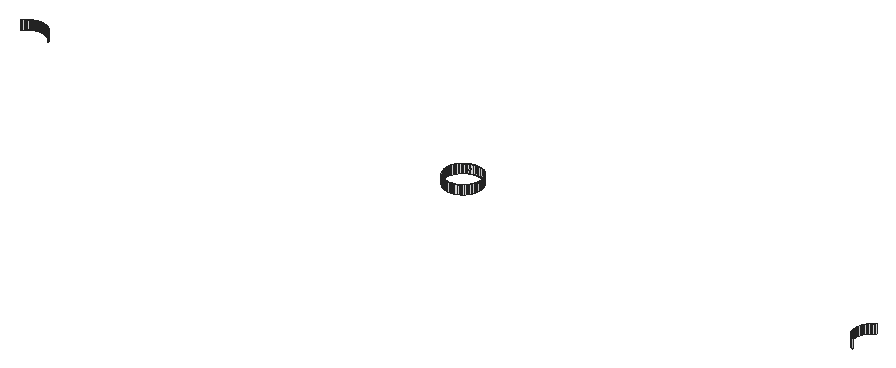
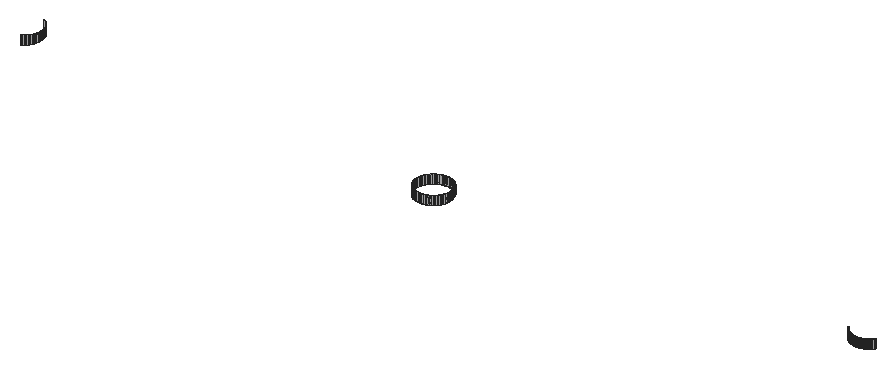
# SketchUp Ruby script. Lengths in inches.
U = 1.inch
M = Sketchup.active_model
def pt(a) = Geom::Point3d.new(a.map { |v| v * U })
def face(e, loops, mat)
  f = e.add_face(loops[0].map { |a| pt(a) })
  loops[1..].each { |l| e.add_face(l.map { |a| pt(a) }).erase! }
  f.material = f.back_material = mat if mat
  f
end
# faces: each face lists its corners as indices into pts; further lists are holes
def faces(e, pts, list, mat = nil) = list.each { |f| face(e, (f[0].is_a?(Array) ? f : [f]).map { |l| l.map { |i| pts[i] } }, mat) }
# xy, xz, yz: faces in a plane at the given z, y or x. An outline is a flat list of corners, or four numbers for a rectangle; further outlines are holes
def ring(l) = l.size == 4 ? [[l[0], l[1]], [l[2], l[1]], [l[2], l[3]], [l[0], l[3]]] : l.each_slice(2).to_a
def flat(e, list, mat, &to3) = list.each { |f| face(e, (f[0].is_a?(Array) ? f : [f]).map { |l| ring(l).map { |u, v| to3.(u, v) } }, mat) }
def xy(e, z, list, mat = nil) = flat(e, list, mat) { |x, y| [x, y, z] }
def xz(e, y, list, mat = nil) = flat(e, list, mat) { |x, z| [x, y, z] }
def yz(e, x, list, mat = nil) = flat(e, list, mat) { |y, z| [x, y, z] }
def lines(e, pts, list) = list.each { |a, b| e.add_line(pt(pts[a]), pt(pts[b])) }
# prism: a flat outline (further loops are holes) pulled along v
def prism(e, loops, v, mat = nil)
  f = face(e, loops, mat); d = Geom::Vector3d.new(v.map { |x| x * U })
  f.pushpull(f.normal.samedirection?(d) ? d.length : -d.length)
end
def box(e, o, s, mat = nil) = prism(e, [[o, [o[0] + s[0], o[1], o[2]], [o[0] + s[0], o[1] + s[1], o[2]], [o[0], o[1] + s[1], o[2]]]], [0, 0, s[2]], mat)
def at(x, y, z, deg = 0) = Geom::Transformation.translation(pt([x, y, z])) * Geom::Transformation.rotation(ORIGIN, Z_AXIS, deg.degrees)
def axes(o, x, y, z) = Geom::Transformation.new([*x, 0, *y, 0, *z, 0, *pt(o).to_a, 1])
def part(name) = M.definitions.add(name)
# library, detail: a bought-in or finely detailed component or shape, given as its bounding box
def library(name, o, s) = part(name).tap { |d| box(d.entities, o, s) }
def detail(e, o, s) = box(e.add_group.entities, o, s)
def put(e, d, t, mat = nil) = e.add_instance(d, t).tap { |i| i.material = mat if mat }
def group(e, t, mat = nil) = e.add_group.tap { |g| g.transformation = t; g.material = mat if mat }.entities
root = M.entities
M.materials.add("[Quartz Light Grey]").color = [251, 251, 252]
xz(root,225.96,[[38.36,111.81,38.38,112.81],[39.62,111.81,39.64,112.81]],"[Quartz Light Grey]")
xz(root,226.01,[[38.52,111.81,38.5625,112.81],[39.4375,111.81,39.48,112.81]],"[Quartz Light Grey]")
xz(root,226.03,[[38.625,111.81,38.65,112.81],[39.35,111.81,39.375,112.81]],"[Quartz Light Grey]")
xz(root,226.04,[[38.6875,111.81,38.73,112.81],[39.27,111.81,39.3125,112.81]],"[Quartz Light Grey]")
xz(root,226.05,[[38.75,111.81,38.77,112.81],[38.77,111.81,38.8125,112.81],[39.1875,111.81,39.23,112.81],[39.23,111.81,39.25,112.81]],"[Quartz Light Grey]")
xz(root,226.06,[[38.85,111.81,38.875,112.81],[38.875,111.81,38.9,112.81],[39.1,111.81,39.125,112.81],[39.125,111.81,39.15,112.81]],"[Quartz Light Grey]")
xz(root,226.0625,[[38.9375,111.81,38.98,112.81],[38.98,111.81,39,112.81],[39,111.81,39.02,112.81],[39.02,111.81,39.0625,112.81]],"[Quartz Light Grey]")
yz(root,85,[[227.96,111.81,228.08,112.81]],"[Quartz Light Grey]")
yz(root,89,[[228.04,111.81,228.17,112.81]],"[Quartz Light Grey]")
yz(root,133,[[227.96,111.81,228.08,112.81]],"[Quartz Light Grey]")
p = [[40.72,225.08,111.81],[40.74,225.05,111.81],[40.74,225.05,112.81],[40.72,225.08,112.81],[40.68,225.15,111.81],[40.6875,225.13,111.81],
  [40.6875,225.13,112.81],[40.68,225.15,112.81],[40.7,225.12,111.81],[40.7,225.12,112.81],[37.35,225.1875,111.81],[37.37,225.22,111.81],
  [37.37,225.22,112.81],[37.35,225.1875,112.81],[37.38,225.24,111.81],[37.38,225.24,112.81],[37.39,225.26,111.81],[37.39,225.26,112.81],
  [40.61,225.26,111.81],[40.62,225.24,111.81],[40.62,225.24,112.81],[40.61,225.26,112.81],[40.63,225.22,111.81],[40.63,225.22,112.81],
  [40.65,225.1875,111.81],[40.65,225.1875,112.81],[37.42,225.29,111.81],[37.42,225.29,112.81],[37.45,225.32,111.81],[37.45,225.32,112.81],
  [37.46,225.34,111.81],[37.46,225.34,112.81],[37.47,225.35,111.81],[37.47,225.35,112.81],[40.53,225.35,111.81],[40.54,225.34,111.81],
  [40.54,225.34,112.81],[40.53,225.35,112.81],[40.55,225.32,111.81],[40.55,225.32,112.81],[40.58,225.29,111.81],[40.58,225.29,112.81],
  [37.5,225.38,111.81],[37.5,225.38,112.81],[37.53,225.42,111.81],[37.53,225.42,112.81],[37.54,225.43,111.81],[37.54,225.43,112.81],
  [37.56,225.45,111.81],[37.56,225.45,112.81],[37.59,225.48,111.81],[37.59,225.48,112.81],[40.41,225.48,111.81],[40.44,225.45,111.81],
  [40.44,225.45,112.81],[40.41,225.48,112.81],[40.46,225.43,111.81],[40.46,225.43,112.81],[40.47,225.42,111.81],[40.47,225.42,112.81],
  [40.5,225.38,111.81],[40.5,225.38,112.81],[37.62,225.51,111.81],[37.62,225.51,112.81],[37.63,225.52,111.81],[37.63,225.52,112.81],
  [37.65,225.54,111.81],[37.65,225.54,112.81],[37.68,225.5625,111.81],[37.68,225.5625,112.81],[40.32,225.5625,111.81],[40.35,225.54,111.81],
  [40.35,225.54,112.81],[40.32,225.5625,112.81],[40.37,225.52,111.81],[40.37,225.52,112.81],[40.38,225.51,111.81],[40.38,225.51,112.81],
  [37.71,225.59,111.81],[37.71,225.59,112.81],[37.73,225.6,111.81],[37.73,225.6,112.81],[37.74,225.62,111.81],[37.74,225.62,112.81],
  [37.77,225.64,111.81],[37.77,225.64,112.81],[37.81,225.67,111.81],[37.81,225.67,112.81],[40.19,225.67,111.81],[40.23,225.64,111.81],
  [40.23,225.64,112.81],[40.19,225.67,112.81],[40.26,225.62,111.81],[40.26,225.62,112.81],[40.27,225.6,111.81],[40.27,225.6,112.81],
  [40.29,225.59,111.81],[40.29,225.59,112.81],[37.82,225.68,111.81],[37.82,225.68,112.81],[37.84,225.69,111.81],[37.84,225.69,112.81],
  [37.875,225.72,111.81],[37.875,225.72,112.81],[37.91,225.74,111.81],[37.91,225.74,112.81],[37.93,225.75,111.81],[37.93,225.75,112.81],
  [40.07,225.75,111.81],[40.09,225.74,111.81],[40.09,225.74,112.81],[40.07,225.75,112.81],[40.125,225.72,111.81],[40.125,225.72,112.81],
  [40.16,225.69,111.81],[40.16,225.69,112.81],[40.18,225.68,111.81],[40.18,225.68,112.81],[37.95,225.76,111.81],[37.95,225.76,112.81],
  [37.98,225.78,111.81],[37.98,225.78,112.81],[38.02,225.8,111.81],[38.02,225.8,112.81],[38.04,225.81,111.81],[38.04,225.81,112.81],
  [38.06,225.83,111.81],[38.06,225.83,112.81],[38.09,225.84,111.81],[38.09,225.84,112.81],[38.13,225.86,111.81],[38.13,225.86,112.81],
  [39.87,225.86,111.81],[39.91,225.84,111.81],[39.91,225.84,112.81],[39.87,225.86,112.81],[39.94,225.83,111.81],[39.94,225.83,112.81],
  [39.96,225.81,111.81],[39.96,225.81,112.81],[39.98,225.8,111.81],[39.98,225.8,112.81],[40.02,225.78,111.81],[40.02,225.78,112.81],
  [40.05,225.76,111.81],[40.05,225.76,112.81],[38.15,225.87,111.81],[38.15,225.87,112.81],[38.17,225.88,111.81],[38.17,225.88,112.81],
  [38.21,225.9,111.81],[38.21,225.9,112.81],[38.24,225.91,111.81],[38.24,225.91,112.81],[38.26,225.92,111.81],[38.26,225.92,112.81],
  [38.28,225.93,111.81],[38.28,225.93,112.81],[38.32,225.94,111.81],[38.32,225.94,112.81],[38.36,225.96,111.81],[38.36,225.96,112.81],
  [39.64,225.96,111.81],[39.68,225.94,111.81],[39.68,225.94,112.81],[39.64,225.96,112.81],[39.72,225.93,111.81],[39.72,225.93,112.81],
  [39.74,225.92,111.81],[39.74,225.92,112.81],[39.76,225.91,111.81],[39.76,225.91,112.81],[39.79,225.9,111.81],[39.79,225.9,112.81],
  [39.83,225.88,111.81],[39.83,225.88,112.81],[39.85,225.87,111.81],[39.85,225.87,112.81],[38.38,225.96,111.81],[38.4,225.97,111.81],
  [38.4,225.97,112.81],[38.38,225.96,112.81],[38.44,225.98,111.81],[38.44,225.98,112.81],[38.48,225.99,111.81],[38.48,225.99,112.81],
  [38.5,226,111.81],[38.5,226,112.81],[38.52,226.01,111.81],[38.52,226.01,112.81],[38.5625,226.01,111.81],[38.6,226.02,111.81],
  [38.6,226.02,112.81],[38.5625,226.01,112.81],[38.625,226.03,111.81],[38.625,226.03,112.81],[38.65,226.03,111.81],[38.6875,226.04,111.81],
  [38.6875,226.04,112.81],[38.65,226.03,112.81],[38.73,226.04,111.81],[38.75,226.05,111.81],[38.75,226.05,112.81],[38.73,226.04,112.81],
  [39.25,226.05,111.81],[39.27,226.04,111.81],[39.27,226.04,112.81],[39.25,226.05,112.81],[39.3125,226.04,111.81],[39.35,226.03,111.81],
  [39.35,226.03,112.81],[39.3125,226.04,112.81],[39.375,226.03,111.81],[39.4,226.02,111.81],[39.4,226.02,112.81],[39.375,226.03,112.81],
  [39.4375,226.01,111.81],[39.4375,226.01,112.81],[39.48,226.01,111.81],[39.5,226,111.81],[39.5,226,112.81],[39.48,226.01,112.81],
  [39.52,225.99,111.81],[39.52,225.99,112.81],[39.56,225.98,111.81],[39.56,225.98,112.81],[39.6,225.97,111.81],[39.6,225.97,112.81],
  [39.62,225.96,111.81],[39.62,225.96,112.81],[38.8125,226.05,111.81],[38.85,226.06,111.81],[38.85,226.06,112.81],[38.8125,226.05,112.81],
  [38.9,226.06,111.81],[38.9375,226.0625,111.81],[38.9375,226.0625,112.81],[38.9,226.06,112.81],[39.0625,226.0625,111.81],[39.1,226.06,111.81],
  [39.1,226.06,112.81],[39.0625,226.0625,112.81],[39.15,226.06,111.81],[39.1875,226.05,111.81],[39.1875,226.05,112.81],[39.15,226.06,112.81],
  [86.48,226.13,111.81],[86.36,226.17,111.81],[86.36,226.17,112.81],[86.48,226.13,112.81],[86.6,226.1,111.81],[86.6,226.1,112.81],
  [86.73,226.08,111.81],[86.73,226.08,112.81],[86.85,226.07,111.81],[86.85,226.07,112.81],[86.98,226.0625,111.81],[86.98,226.0625,112.81],
  [87.1,226.07,111.81],[87.1,226.07,112.81],[87.23,226.08,111.81],[87.23,226.08,112.81],[87.35,226.09,111.81],[87.35,226.09,112.81],
  [87.48,226.12,111.81],[87.48,226.12,112.81],[87.6,226.15,111.81],[87.6,226.15,112.81],[86.24,226.21,111.81],[86.13,226.26,111.81],
  [86.13,226.26,112.81],[86.24,226.21,112.81],[87.72,226.2,111.81],[87.72,226.2,112.81],[87.83,226.24,111.81],[87.83,226.24,112.81],
  [87.94,226.3,111.81],[87.94,226.3,112.81],[86.02,226.32,111.81],[85.91,226.39,111.81],[85.91,226.39,112.81],[86.02,226.32,112.81],
  [88.05,226.36,111.81],[88.05,226.36,112.81],[134.02,226.32,111.81],[133.91,226.39,111.81],[133.91,226.39,112.81],[134.02,226.32,112.81],
  [134.13,226.26,111.81],[134.13,226.26,112.81],[85.81,226.46,111.81],[85.81,226.46,112.81],[88.16,226.43,111.81],[88.16,226.43,112.81],
  [88.26,226.51,111.81],[88.26,226.51,112.81],[133.81,226.46,111.81],[133.81,226.46,112.81],[85.71,226.54,111.81],[85.62,226.62,111.81],
  [85.62,226.62,112.81],[85.71,226.54,112.81],[88.35,226.59,111.81],[88.35,226.59,112.81],[133.71,226.54,111.81],[133.62,226.62,111.81],
  [133.62,226.62,112.81],[133.71,226.54,112.81],[85.53,226.71,111.81],[85.53,226.71,112.81],[88.44,226.68,111.81],[88.44,226.68,112.81],
  [133.53,226.71,111.81],[133.53,226.71,112.81],[85.45,226.8,111.81],[85.45,226.8,112.81],[88.53,226.77,111.81],[88.53,226.77,112.81],
  [133.45,226.8,111.81],[133.45,226.8,112.81],[85.37,226.9,111.81],[85.37,226.9,112.81],[88.61,226.87,111.81],[88.61,226.87,112.81],
  [133.37,226.9,111.81],[133.37,226.9,112.81],[85.3,227.01,111.81],[85.3,227.01,112.81],[88.68,226.97,111.81],[88.68,226.97,112.81],
  [133.3,227.01,111.81],[133.3,227.01,112.81],[85.24,227.12,111.81],[85.24,227.12,112.81],[88.74,227.08,111.81],[88.74,227.08,112.81],
  [133.24,227.12,111.81],[133.24,227.12,112.81],[85.18,227.23,111.81],[85.18,227.23,112.81],[88.8,227.19,111.81],[88.8,227.19,112.81],
  [133.18,227.23,111.81],[133.18,227.23,112.81],[85.13,227.35,111.81],[85.13,227.35,112.81],[88.85,227.31,111.81],[88.85,227.31,112.81],
  [133.13,227.35,111.81],[133.13,227.35,112.81],[85.09,227.47,111.81],[85.09,227.47,112.81],[88.9,227.42,111.81],[88.9,227.42,112.81],
  [133.09,227.47,111.81],[133.09,227.47,112.81],[88.93,227.54,111.81],[88.93,227.54,112.81],[85.06,227.59,111.81],[85.06,227.59,112.81],
  [88.96,227.67,111.81],[88.96,227.67,112.81],[133.06,227.59,111.81],[133.06,227.59,112.81],[85.03,227.71,111.81],[85.03,227.71,112.81],
  [133.03,227.71,111.81],[133.03,227.71,112.81],[85.01,227.83,111.81],[85.01,227.83,112.81],[88.98,227.79,111.81],[88.98,227.79,112.81],
  [133.01,227.83,111.81],[133.01,227.83,112.81],[85,227.96,111.81],[85,227.96,112.81],[88.99,227.92,111.81],[88.99,227.92,112.81],
  [133,227.96,111.81],[133,227.96,112.81],[89,228.04,111.81],[89,228.04,112.81],[85,228.08,111.81],[85.01,228.21,111.81],
  [85.01,228.21,112.81],[85,228.08,112.81],[133,228.08,111.81],[133.01,228.21,111.81],[133.01,228.21,112.81],[133,228.08,112.81],
  [85.02,228.33,111.81],[85.02,228.33,112.81],[88.99,228.29,111.81],[89,228.17,111.81],[89,228.17,112.81],[88.99,228.29,112.81],
  [133.02,228.33,111.81],[133.02,228.33,112.81],[85.04,228.46,111.81],[85.04,228.46,112.81],[88.97,228.42,111.81],[88.97,228.42,112.81],
  [133.04,228.46,111.81],[133.04,228.46,112.81],[88.94,228.54,111.81],[88.94,228.54,112.81],[85.07,228.58,111.81],[85.07,228.58,112.81],
  [88.91,228.66,111.81],[88.91,228.66,112.81],[133.07,228.58,111.81],[133.07,228.58,112.81],[85.1,228.7,111.81],[85.1,228.7,112.81],
  [133.1,228.7,111.81],[133.1,228.7,112.81],[85.15,228.82,111.81],[85.15,228.82,112.81],[88.87,228.78,111.81],[88.87,228.78,112.81],
  [133.15,228.82,111.81],[133.15,228.82,112.81],[85.2,228.93,111.81],[85.2,228.93,112.81],[88.82,228.89,111.81],[88.82,228.89,112.81],
  [133.2,228.93,111.81],[133.2,228.93,112.81],[85.26,229.05,111.81],[85.26,229.05,112.81],[88.76,229.01,111.81],[88.76,229.01,112.81],
  [133.26,229.05,111.81],[133.26,229.05,112.81],[85.32,229.15,111.81],[85.32,229.15,112.81],[88.7,229.12,111.81],[88.7,229.12,112.81],
  [133.32,229.15,111.81],[133.32,229.15,112.81],[88.63,229.22,111.81],[88.63,229.22,112.81],[85.39,229.26,111.81],[85.39,229.26,112.81],
  [88.55,229.32,111.81],[88.55,229.32,112.81],[133.39,229.26,111.81],[133.39,229.26,112.81],[85.47,229.35,111.81],[85.47,229.35,112.81],
  [88.47,229.42,111.81],[88.47,229.42,112.81],[133.47,229.35,111.81],[133.47,229.35,112.81],[85.56,229.45,111.81],[85.56,229.45,112.81],
  [85.65,229.54,111.81],[85.65,229.54,112.81],[88.38,229.51,111.81],[88.38,229.51,112.81],[133.56,229.45,111.81],[133.56,229.45,112.81],
  [133.65,229.54,111.81],[133.65,229.54,112.81],[85.74,229.62,111.81],[85.74,229.62,112.81],[88.29,229.59,111.81],[88.29,229.59,112.81],
  [133.74,229.62,111.81],[133.74,229.62,112.81],[85.84,229.69,111.81],[85.84,229.69,112.81],[88.19,229.67,111.81],[88.19,229.67,112.81],
  [133.84,229.69,111.81],[133.84,229.69,112.81],[85.95,229.76,111.81],[85.95,229.76,112.81],[87.98,229.8,111.81],[88.09,229.74,111.81],
  [88.09,229.74,112.81],[87.98,229.8,112.81],[133.95,229.76,111.81],[133.95,229.76,112.81],[86.06,229.83,111.81],[86.06,229.83,112.81],
  [86.17,229.88,111.81],[86.17,229.88,112.81],[87.87,229.86,111.81],[87.87,229.86,112.81],[134.06,229.83,111.81],[134.06,229.83,112.81],
  [86.28,229.93,111.81],[86.28,229.93,112.81],[86.4,229.97,111.81],[86.4,229.97,112.81],[87.64,229.96,111.81],[87.76,229.91,111.81],
  [87.76,229.91,112.81],[87.64,229.96,112.81],[86.52,230.01,111.81],[86.52,230.01,112.81],[86.65,230.03,111.81],[86.65,230.03,112.81],
  [86.77,230.05,111.81],[86.77,230.05,112.81],[86.9,230.06,111.81],[86.9,230.06,112.81],[87.15,230.06,111.81],[87.27,230.04,111.81],
  [87.27,230.04,112.81],[87.15,230.06,112.81],[87.4,230.02,111.81],[87.4,230.02,112.81],[87.52,229.99,111.81],[87.52,229.99,112.81],
  [87.02,230.0625,111.81],[87.02,230.0625,112.81]]
faces(root,p,[[0,1,2,3],[4,5,6,7],[5,8,9,6],[8,0,3,9],[10,11,12,13],[11,14,15,12],[14,16,17,15],[18,19,20,21],
  [19,22,23,20],[22,24,25,23],[24,4,7,25],[16,26,27,17],[26,28,29,27],[28,30,31,29],[30,32,33,31],[34,35,36,37],
  [35,38,39,36],[38,40,41,39],[40,18,21,41],[32,42,43,33],[42,44,45,43],[44,46,47,45],[46,48,49,47],[48,50,51,49],
  [52,53,54,55],[53,56,57,54],[56,58,59,57],[58,60,61,59],[60,34,37,61],[50,62,63,51],[62,64,65,63],[64,66,67,65],
  [66,68,69,67],[70,71,72,73],[71,74,75,72],[74,76,77,75],[76,52,55,77],[68,78,79,69],[78,80,81,79],[80,82,83,81],
  [82,84,85,83],[84,86,87,85],[88,89,90,91],[89,92,93,90],[92,94,95,93],[94,96,97,95],[96,70,73,97],[86,98,99,87],
  [98,100,101,99],[100,102,103,101],[102,104,105,103],[104,106,107,105],[108,109,110,111],[109,112,113,110],[112,114,115,113],[114,116,117,115],
  [116,88,91,117],[106,118,119,107],[118,120,121,119],[120,122,123,121],[122,124,125,123],[124,126,127,125],[126,128,129,127],[128,130,131,129],
  [132,133,134,135],[133,136,137,134],[136,138,139,137],[138,140,141,139],[140,142,143,141],[142,144,145,143],[144,108,111,145],[130,146,147,131],
  [146,148,149,147],[148,150,151,149],[150,152,153,151],[152,154,155,153],[154,156,157,155],[156,158,159,157],[158,160,161,159],[162,163,164,165],
  [163,166,167,164],[166,168,169,167],[168,170,171,169],[170,172,173,171],[172,174,175,173],[174,176,177,175],[176,132,135,177],[178,179,180,181],
  [179,182,183,180],[182,184,185,183],[184,186,187,185],[186,188,189,187],[190,191,192,193],[191,194,195,192],[196,197,198,199],[200,201,202,203],
  [204,205,206,207],[208,209,210,211],[212,213,214,215],[213,216,217,214],[218,219,220,221],[219,222,223,220],[222,224,225,223],[224,226,227,225],
  [226,228,229,227],[230,231,232,233],[234,235,236,237],[238,239,240,241],[242,243,244,245],[246,247,248,249],[250,246,249,251],[252,250,251,253],
  [254,252,253,255],[256,254,255,257],[258,256,257,259],[260,258,259,261],[262,260,261,263],[264,262,263,265],[266,264,265,267],[268,269,270,271],
  [247,268,271,248],[272,266,267,273],[274,272,273,275],[276,274,275,277],[278,279,280,281],[269,278,281,270],[282,276,277,283],[284,285,286,287],
  [288,284,287,289],[279,290,291,280],[292,282,283,293],[294,292,293,295],[285,296,297,286],[298,299,300,301],[290,298,301,291],[302,294,295,303],
  [304,305,306,307],[296,304,307,297],[299,308,309,300],[310,302,303,311],[305,312,313,306],[308,314,315,309],[316,310,311,317],[312,318,319,313],
  [314,320,321,315],[322,316,317,323],[318,324,325,319],[320,326,327,321],[328,322,323,329],[324,330,331,325],[326,332,333,327],[334,328,329,335],
  [330,336,337,331],[332,338,339,333],[340,334,335,341],[336,342,343,337],[338,344,345,339],[346,340,341,347],[342,348,349,343],[344,350,351,345],
  [352,346,347,353],[348,354,355,349],[356,352,353,357],[350,358,359,351],[360,356,357,361],[354,362,363,355],[358,364,365,359],[362,366,367,363],
  [364,368,369,365],[370,360,361,371],[366,372,373,367],[368,374,375,369],[376,370,371,377],[372,378,379,373],[380,376,377,381],[382,383,384,385],
  [386,387,388,389],[383,390,391,384],[392,393,394,395],[387,396,397,388],[390,398,399,391],[400,392,395,401],[396,402,403,397],[404,400,401,405],
  [398,406,407,399],[408,404,405,409],[402,410,411,403],[406,412,413,407],[410,414,415,411],[412,416,417,413],[418,408,409,419],[414,420,421,415],
  [416,422,423,417],[424,418,419,425],[420,426,427,421],[422,428,429,423],[430,424,425,431],[426,432,433,427],[428,434,435,429],[436,430,431,437],
  [432,438,439,433],[440,436,437,441],[434,442,443,435],[444,440,441,445],[438,446,447,439],[442,448,449,443],[450,444,445,451],[446,452,453,447],
  [448,454,455,449],[454,456,457,455],[458,450,451,459],[452,460,461,453],[460,462,463,461],[456,464,465,457],[466,458,459,467],[462,468,469,463],
  [464,470,471,465],[472,466,467,473],[468,474,475,469],[470,476,477,471],[478,479,480,481],[479,472,473,480],[474,482,483,475],[476,484,485,477],
  [484,486,487,485],[488,478,481,489],[482,490,491,483],[486,492,493,487],[492,494,495,493],[496,497,498,499],[497,488,489,498],[494,500,501,495],
  [500,502,503,501],[502,504,505,503],[504,506,507,505],[508,509,510,511],[509,512,513,510],[512,514,515,513],[514,496,499,515],[506,516,517,507],
  [516,508,511,517]],"[Quartz Light Grey]")
